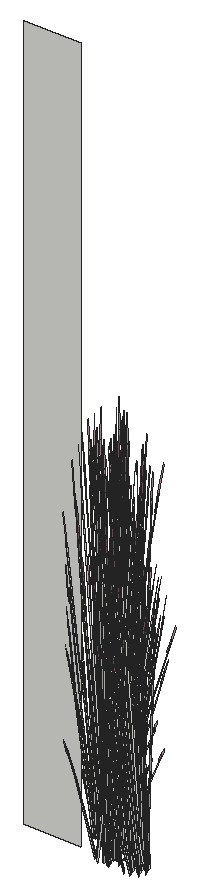
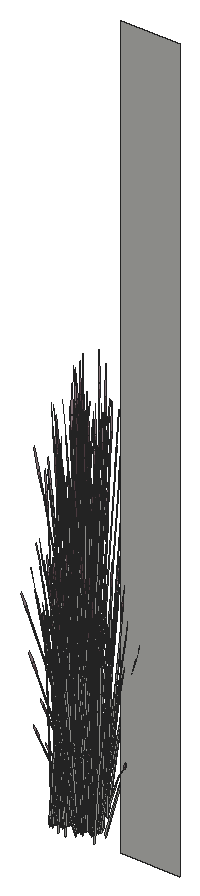
# SketchUp Ruby script. Lengths in inches.
U = 1.inch
M = Sketchup.active_model
def pt(a) = Geom::Point3d.new(a.map { |v| v * U })
def face(e, loops, mat)
  f = e.add_face(loops[0].map { |a| pt(a) })
  loops[1..].each { |l| e.add_face(l.map { |a| pt(a) }).erase! }
  f.material = f.back_material = mat if mat
  f
end
# faces: each face lists its corners as indices into pts; further lists are holes
def faces(e, pts, list, mat = nil) = list.each { |f| face(e, (f[0].is_a?(Array) ? f : [f]).map { |l| l.map { |i| pts[i] } }, mat) }
# xy, xz, yz: faces in a plane at the given z, y or x. An outline is a flat list of corners, or four numbers for a rectangle; further outlines are holes
def ring(l) = l.size == 4 ? [[l[0], l[1]], [l[2], l[1]], [l[2], l[3]], [l[0], l[3]]] : l.each_slice(2).to_a
def flat(e, list, mat, &to3) = list.each { |f| face(e, (f[0].is_a?(Array) ? f : [f]).map { |l| ring(l).map { |u, v| to3.(u, v) } }, mat) }
def xy(e, z, list, mat = nil) = flat(e, list, mat) { |x, y| [x, y, z] }
def xz(e, y, list, mat = nil) = flat(e, list, mat) { |x, z| [x, y, z] }
def yz(e, x, list, mat = nil) = flat(e, list, mat) { |y, z| [x, y, z] }
def lines(e, pts, list) = list.each { |a, b| e.add_line(pt(pts[a]), pt(pts[b])) }
# prism: a flat outline (further loops are holes) pulled along v
def prism(e, loops, v, mat = nil)
  f = face(e, loops, mat); d = Geom::Vector3d.new(v.map { |x| x * U })
  f.pushpull(f.normal.samedirection?(d) ? d.length : -d.length)
end
def box(e, o, s, mat = nil) = prism(e, [[o, [o[0] + s[0], o[1], o[2]], [o[0] + s[0], o[1] + s[1], o[2]], [o[0], o[1] + s[1], o[2]]]], [0, 0, s[2]], mat)
def at(x, y, z, deg = 0) = Geom::Transformation.translation(pt([x, y, z])) * Geom::Transformation.rotation(ORIGIN, Z_AXIS, deg.degrees)
def axes(o, x, y, z) = Geom::Transformation.new([*x, 0, *y, 0, *z, 0, *pt(o).to_a, 1])
def part(name) = M.definitions.add(name)
# library, detail: a bought-in or finely detailed component or shape, given as its bounding box
def library(name, o, s) = part(name).tap { |d| box(d.entities, o, s) }
def detail(e, o, s) = box(e.add_group.entities, o, s)
def put(e, d, t, mat = nil) = e.add_instance(d, t).tap { |i| i.material = mat if mat }
def group(e, t, mat = nil) = e.add_group.tap { |g| g.transformation = t; g.material = mat if mat }.entities
root = M.entities
M.materials.add("LightPink_Translucent").color = [144, 107, 117]
M.materials["LightPink_Translucent"].alpha = 0.75
c1 = part("blade")
p = [[2.15,0.21,22],[0,0.17,0],[0.09,0.45,0],[2.18,0.31,22],[2.29,0.31,22],[0.38,0.45,0],
  [2.48,0.24,33],[2.49,0.24,33],[2.48,0.22,33]]
faces(c1.entities,p,[[0,1,2,3],[4,5,2,3],[6,3,4,7],[8,0,3,6]])
c2 = part("seeds")
p = [[0.3,-0.1,1.38],[-0.01,-0.03,1.59],[-0.01,-0.03,0.03],[0.14,-0.07,-0.07],[0.29,-0.03,3],[0.15,0.01,3.11]]
faces(c2.entities,p,[[0,1,2,3],[1,0,4,5]],"LightPink_Translucent")
c3 = part("blade with seeds")
put(c3.entities,c1,at(0,0,0))
put(c3.entities,c2,axes([2.4,0.25,30.99],[1.5799,-0.05474,1.17369],[-0.12525,1.92788,0.29478],[-0.07173,-0.02425,1.56792]))
xz(root,652.9,[[321.57,621,330.57,735]])
put(root,c3,axes([334.34,651.43,623.6],[0.12246,-0.09864,1.71376],[0.1031,0.45582,0.13857],[-0.19225,0.10302,0.73262]))
put(root,c3,axes([333.96,652.2,622.31],[0.12266,0.03828,1.43002],[0.07906,0.39104,-0.30754],[-0.16661,0.0732,0.61141]))
put(root,c3,axes([335.04,650.95,623.07],[0.10032,-0.06746,1.77064],[0.0346,0.47103,0.13857],[-0.2173,0.0625,0.63284]))
put(root,c3,axes([333.96,651.27,624.4375],[-0.05763,0.06055,1.74944],[0.0049,0.44239,-0.27667],[-0.13211,0.05753,0.14031]))
put(root,c3,axes([334.15,651.01,624.25],[-0.29332,-0.1301,-0.35414],[0.08555,-0.37955,0.4572],[-0.11809,0.0348,0.87481]))
put(root,c3,axes([333.32,651.71,624.43],[0.04504,0.01251,1.77383],[0.13934,0.41205,-0.16761],[-0.0922,0.10815,0.31391]))
put(root,c3,axes([334.35,651.21,624.4],[-0.09562,0.42421,-0.51099],[-0.32782,-0.1454,-0.3958],[-0.13199,0.0389,0.97773]))
put(root,c3,axes([334.18,651.18,621.22],[0.00895,0.0735,1.76342],[-0.18044,0.38382,-0.26939],[-0.12817,-0.01935,0.30037]))
put(root,c3,axes([333.7,653.02,622.49],[0.14709,-0.21136,1.1486],[0.05804,0.3346,0.84392],[-0.1063,0.05991,0.25299]))
put(root,c3,axes([334.22,650.97,624.46],[0.09971,-0.42522,0.48003],[0.32782,0.1454,0.3958],[-0.12892,0.02555,0.9933]))
put(root,c3,axes([334.33,650.84,624.76],[0.17758,0.42229,-0.1216],[-0.31518,0.20752,-0.67495],[-0.13282,0.05572,1.02557]))
put(root,c3,axes([334.19,650.85,624.45],[-0.12963,-0.31798,0.0643],[0.23638,-0.15564,0.50621],[-0.1042,0.03071,0.77189]))
put(root,c3,axes([334.78,651.73,623.6],[0.08815,-0.14329,1.71376],[0.22258,0.38678,0.13857],[-0.15267,0.17614,0.73262]))
put(root,c3,axes([334.25,652.11,624.25],[-0.30722,0.06665,-0.35414],[-0.08112,-0.381,0.4572],[-0.08804,0.10234,0.87481]))
put(root,c3,axes([334.09,653.24,621.22],[0.04734,0.04659,1.76342],[0.08027,0.4317,-0.26939],[-0.10492,0.09206,0.30037]))
put(root,c3,axes([334.29,652.03,624.46],[-0.08753,-0.42921,0.48003],[0.34336,-0.07449,0.3958],[-0.1012,0.10094,0.9933]))
put(root,c3,axes([334.23,651.94,624.45],[-0.2423,-0.19613,0.0643],[0.14107,-0.2793,0.50621],[-0.07768,0.0903,0.77189]))
put(root,c3,axes([334.72,652.09,623.6],[0.06572,-0.16029,1.71376],[0.27569,0.33172,0.13857],[-0.12437,0.20675,0.73262]))
put(root,c3,axes([334.46,650.97,624.78],[0.29332,0.1301,0.35414],[-0.08555,0.37955,-0.4572],[-0.11809,0.0348,0.87481]))
put(root,c3,axes([334.51,652.15,624.4],[0.09067,0.42583,-0.51099],[-0.34336,0.07449,-0.3958],[-0.0984,0.11438,0.97773]))
put(root,c3,axes([335.36,651.85,621.78],[-0.36714,-0.07646,-0.62353],[0.07747,-0.47163,-0.16365],[-0.10956,-0.05715,1.37633]))
put(root,c3,axes([334.88,652.74,621.74],[-0.33032,-0.23318,-0.49651],[0.19744,-0.41812,0],[-0.07523,-0.05311,1.57504]))
put(root,c3,axes([334.35,651.85,624.76],[0.32648,0.25715,-0.1216],[-0.18809,0.3724,-0.67495],[-0.09224,0.12945,1.02557]))
put(root,c3,axes([335.08,653.02,622.1],[-0.22066,0.46731,0],[-0.36918,-0.26061,-0.51607],[-0.08408,-0.05936,1.63711]))
put(root,c3,axes([333.81,652.96,625.37],[0.31145,0.12449,-0.06488],[-0.0958,0.38314,-0.29416],[-0.05094,0.05817,0.97024]))
put(root,c3,axes([334.5,651.88,624.78],[0.30722,-0.06665,0.35414],[0.08112,0.381,-0.4572],[-0.08804,0.10234,0.87481]))
put(root,c3,axes([335.78,651.92,622.39],[-0.35635,0.30962,-0.29095],[-0.23697,-0.43749,-0.50002],[-0.08792,-0.04443,1.59708]))
put(root,c3,axes([334.8,652.89,624.46],[-0.25132,-0.3182,0.48003],[0.2669,-0.27442,0.3958],[-0.04636,0.14929,0.9933]))
put(root,c3,axes([334.97,652.57,621.75],[-0.08291,-0.40636,-0.30978],[0.32928,-0.11539,0.30978],[-0.06638,-0.04686,1.38974]))
put(root,c3,axes([334.7,652.86,624.45],[-0.29004,-0.02173,0.0643],[0.00795,-0.32812,0.50621],[-0.03035,0.12569,0.77189]))
put(root,c3,axes([336.02,652.25,621.78],[-0.23773,0.35053,-0.62353],[-0.29532,-0.31785,-0.16365],[-0.09526,0.08744,1.37633]))
put(root,c3,axes([336.18,652.06,622.1875],[-0.34464,-0.37536,-0.25192],[0.29,-0.42149,0.5513],[-0.0928,0.04391,1.68216]))
put(root,c3,axes([336.01,651.98,621.93],[-0.38326,0.02879,-0.44739],[-0.03466,-0.47788,0.21531],[-0.06861,0.04843,1.43643]))
put(root,c3,axes([335.27,652.78,622.2],[0.33032,0.23318,0.49651],[-0.19744,0.41812,0],[-0.07523,-0.05311,1.57504]))
put(root,c3,axes([335.75,652.05,622.34],[-0.06809,0.4162,0.1448],[-0.33266,-0.07225,-0.41347],[-0.06054,-0.04274,1.26744]))
put(root,c3,axes([336.41,653.21,621.74],[-0.33032,0.23318,-0.49651],[-0.19744,-0.41812,0],[-0.07523,0.05311,1.57504]))
put(root,c3,axes([336.43,653.09,621.92],[-0.21791,-0.46895,-0.05142],[0.36918,-0.26061,0.51607],[-0.09097,0.04465,1.6363]))
put(root,c3,axes([336.33,653.03,621.75],[-0.32928,-0.11539,-0.30978],[0.08291,-0.40636,0.30978],[-0.06638,0.04686,1.38974]))
put(root,c3,axes([334.92,652.64,624.78],[0.23881,-0.24554,0.35414],[0.22606,0.28036,-0.4572],[-0.0344,0.14245,0.87481]))
put(root,c3,axes([336.52,651.29,622.57],[-0.00964,-0.43909,1.41272],[0.43635,0.11382,0.59816],[-0.1032,0.24027,1.3335]))
put(root,c3,axes([336.27,651.85,622.39],[0.04113,0.53214,-0.29095],[-0.42835,0.03218,-0.50002],[-0.07543,0.07088,1.59708]))
put(root,c3,axes([335.64,651.66,622.09],[0.44609,0.09826,0.45755],[-0.09078,0.55493,0.17955],[-0.06519,-0.05359,1.58856]))
put(root,c3,axes([335.52,651.55,622.44],[-0.17124,0.42022,0.44739],[-0.35581,-0.20224,-0.21531],[0,-0.09687,1.43643]))
put(root,c3,axes([335.4,652.54,622.2],[0.37926,-0.12378,0.17642],[0.09365,0.46065,0.35086],[-0.03382,-0.06712,1.60407]))
put(root,c3,axes([335.89,652.61,621.92],[-0.35581,-0.20937,0],[0.17124,-0.43505,0],[0,0,1.62707]))
put(root,c3,axes([336.71,653.14,622.1],[0.22066,0.46731,0],[-0.36918,0.26061,-0.51607],[-0.08408,0.05936,1.63711]))
put(root,c3,axes([338.8,651.43,623.1],[0.12246,-0.09864,1.71376],[0.1031,0.45582,0.13857],[-0.19225,0.10302,0.73262]))
put(root,c3,axes([336.53,652.57,622.2],[0.10196,-0.46348,0.17642],[0.3731,0.13116,0.35086],[-0.06445,0.00226,1.60407]))
put(root,c3,axes([336.35,651.95,622.34],[0.26075,0.2802,0.1448],[-0.2175,0.31612,-0.41347],[-0.06054,0.04274,1.26744]))
put(root,c3,axes([338.42,652.2,621.81],[0.12266,0.03828,1.43002],[0.07906,0.39104,-0.30754],[-0.16661,0.0732,0.61141]))
put(root,c3,axes([336.26,651.61,622.02],[-0.32829,-0.4014,-0.06131],[0.32849,-0.40164,0],[-0.01146,-0.01402,1.75571]))
put(root,c3,axes([336.35,651.75,622.44],[0.38326,-0.02879,0.44739],[0.03466,0.47788,-0.21531],[-0.06861,0.04843,1.43643]))
put(root,c3,axes([339.5,650.95,622.57],[0.10032,-0.06746,1.77064],[0.0346,0.47103,0.13857],[-0.2173,0.0625,0.63284]))
put(root,c3,axes([336.44,652.85,622.05],[0.44186,0.15158,0.30756],[-0.11054,0.54181,-0.36492],[-0.07313,0.06781,1.64885]))
put(root,c3,axes([336.63,652.82,622.2],[0.33032,-0.23318,0.49651],[0.19744,0.41812,0],[-0.07523,0.05311,1.57504]))
put(root,c3,axes([335.97,652.43,621.93],[-0.11516,-0.40207,0],[0.32884,-0.1408,0],[0,0,1.54371]))
put(root,c3,axes([338.42,651.27,623.9375],[-0.05763,0.06055,1.74944],[0.0049,0.44239,-0.27667],[-0.13211,0.05753,0.14031]))
put(root,c3,axes([338.61,651.01,623.75],[-0.29332,-0.1301,-0.35414],[0.08555,-0.37955,0.4572],[-0.11809,0.0348,0.87481]))
put(root,c3,axes([336.43,651.64,621.93],[-0.17124,0.42022,-0.44739],[-0.35581,-0.20224,0.21531],[0,0.09687,1.43643]))
put(root,c3,axes([337.78,651.71,623.93],[0.04504,0.01251,1.77383],[0.13934,0.41205,-0.16761],[-0.0922,0.10815,0.31391]))
put(root,c3,axes([337.11,651.38,622.2],[-0.2773,-0.3397,0.17642],[0.27945,-0.32949,0.35086],[-0.03063,0.06937,1.60407]))
put(root,c3,axes([338.81,651.21,623.9],[-0.09562,0.42421,-0.51099],[-0.32782,-0.1454,-0.3958],[-0.13199,0.0389,0.97773]))
put(root,c3,axes([336.15,651.1875,621.93],[0,-0.53961,0],[0.44133,0,0],[0,0,1.79456]))
put(root,c3,axes([336.37,651.4,622.02],[0,0.53934,-0.05637],[-0.44133,0,0],[0,0.01695,1.79368]))
put(root,c3,axes([338.64,651.18,620.72],[0.00895,0.0735,1.76342],[-0.18044,0.38382,-0.26939],[-0.12817,-0.01935,0.30037]))
put(root,c3,axes([335.59,653.05,624.78],[0.1064,-0.35863,0.35414],[0.31043,0.1046,-0.4572],[0.02846,0.14439,0.87481]))
put(root,c3,axes([335.43,650.15,622.2],[-0.10196,0.46348,0.17642],[-0.3731,-0.13116,0.35086],[0.06445,-0.00226,1.60407]))
put(root,c3,axes([336.16,652.45,622.02],[0.15345,0.53576,-0.06012],[-0.43845,0.18773,0],[0.00536,0.01871,1.72173]))
put(root,c3,axes([338.16,653.02,621.99],[0.14709,-0.21136,1.1486],[0.05804,0.3346,0.84392],[-0.1063,0.05991,0.25299]))
put(root,c3,axes([337.43,651.74,621.92],[-0.44111,-0.00373,-0.04976],[0,-0.52122,0.49943],[-0.01386,0.11865,1.58352]))
put(root,c3,axes([338.68,650.97,623.96],[0.09971,-0.42522,0.48003],[0.32782,0.1454,0.3958],[-0.12892,0.02555,0.9933]))
put(root,c3,axes([338.79,650.84,624.26],[0.17758,0.42229,-0.1216],[-0.31518,0.20752,-0.67495],[-0.13282,0.05572,1.02557]))
put(root,c3,axes([339.875,651.43,623.19],[0.12246,-0.09864,1.71376],[0.1031,0.45582,0.13857],[-0.19225,0.10302,0.73262]))
put(root,c3,axes([336.5625,650.18,622.2],[-0.37926,0.12378,0.17642],[-0.09365,-0.46065,0.35086],[0.03382,0.06712,1.60407]))
put(root,c3,axes([338.65,650.85,623.95],[-0.12963,-0.31798,0.0643],[0.23638,-0.15564,0.50621],[-0.1042,0.03071,0.77189]))
put(root,c3,axes([339.25,651.73,623.1],[0.08815,-0.14329,1.71376],[0.22258,0.38678,0.13857],[-0.15267,0.17614,0.73262]))
put(root,c3,axes([338.71,652.11,623.75],[-0.30722,0.06665,-0.35414],[-0.08112,-0.381,0.4572],[-0.08804,0.10234,0.87481]))
put(root,c3,axes([339.49,652.2,621.91],[0.12266,0.03828,1.43002],[0.07906,0.39104,-0.30754],[-0.16661,0.0732,0.61141]))
put(root,c3,axes([336.01,654.32,625.37],[0.2439,-0.26754,-0.06488],[0.22348,0.29302,-0.29416],[0.01573,0.08303,0.97024]))
put(root,c3,axes([335.94,650.85,622.09],[-0.29264,0.42323,0.45755],[-0.34767,-0.3736,0.17955],[0.07055,-0.04224,1.58856]))
put(root,c3,axes([338.55,653.24,620.72],[0.04734,0.04659,1.76342],[0.08027,0.4317,-0.26939],[-0.10492,0.09206,0.30037]))
put(root,c3,axes([336.44,651.52,621.9375],[0.24637,0.30123,0],[-0.24637,0.30123,0],[0,0,1.69266]))
put(root,c3,axes([336.4375,651.16,622.44],[0.17124,-0.42022,0.44739],[0.35581,0.20224,-0.21531],[0,0.09687,1.43643]))
put(root,c3,axes([336.29,652.62,621.93],[0.35581,0.20937,0],[-0.17124,0.43505,0],[0,0,1.74954]))
put(root,c3,axes([340.58,650.95,622.66],[0.10032,-0.06746,1.77064],[0.0346,0.47103,0.13857],[-0.2173,0.0625,0.63284]))
put(root,c3,axes([338.75,652.03,623.96],[-0.08753,-0.42921,0.48003],[0.34336,-0.07449,0.3958],[-0.1012,0.10094,0.9933]))
put(root,c3,axes([336.32,651.0625,622.11],[-0.44609,-0.09826,0.49198],[0.09078,-0.55493,0.19306],[0.06519,0.05359,1.70813]))
put(root,c3,axes([337.34,651.82,621.75],[-0.24637,0.29097,-0.30978],[-0.24637,-0.29097,0.30978],[0,0.09372,1.38974]))
put(root,c3,axes([338.6875,651.94,623.95],[-0.2423,-0.19613,0.0643],[0.14107,-0.2793,0.50621],[-0.07768,0.0903,0.77189]))
put(root,c3,axes([336.63,651.77,621.82],[0.12941,0.42699,-0.69212],[-0.37279,0.15378,-0.18165],[0.0143,0.14459,1.52773]))
put(root,c3,axes([336.45,651.31,621.93],[0.39487,0,0],[0,0.48281,0],[0,0,1.78407]))
put(root,c3,axes([339.5,651.27,624.03],[-0.05763,0.06055,1.74944],[0.0049,0.44239,-0.27667],[-0.13211,0.05753,0.14031]))
put(root,c3,axes([336.07,650.78,622.44],[-0.21202,-0.39143,0.44739],[0.32115,-0.27564,-0.21531],[0.06861,0.04843,1.43643]))
put(root,c3,axes([339.18,652.09,623.1],[0.06572,-0.16029,1.71376],[0.27569,0.33172,0.13857],[-0.12437,0.20675,0.73262]))
put(root,c3,axes([336.59,651.26,622.34],[0.32884,-0.136,0.1448],[0.11516,0.38837,-0.41347],[0,0.08547,1.26744]))
put(root,c3,axes([339.69,651.01,623.84],[-0.29332,-0.1301,-0.35414],[0.08555,-0.37955,0.4572],[-0.11809,0.0348,0.87481]))
put(root,c3,axes([338.92,650.97,624.28],[0.29332,0.1301,0.35414],[-0.08555,0.37955,-0.4572],[-0.11809,0.0348,0.87481]))
put(root,c3,axes([336.47,651.29,622.39],[0.39748,0.22252,-0.29095],[-0.19139,0.46966,-0.50002],[0.01249,0.11531,1.59708]))
put(root,c3,axes([338.97,652.15,623.9],[0.09067,0.42583,-0.51099],[-0.34336,0.07449,-0.3958],[-0.0984,0.11438,0.97773]))
put(root,c3,axes([338.86,651.71,624.03],[0.04504,0.01251,1.77383],[0.13934,0.41205,-0.16761],[-0.0922,0.10815,0.31391]))
put(root,c3,axes([339.89,651.21,624],[-0.09562,0.42421,-0.51099],[-0.32782,-0.1454,-0.3958],[-0.13199,0.0389,0.97773]))
put(root,c3,axes([339.82,651.85,621.28],[-0.36714,-0.07646,-0.62353],[0.07747,-0.47163,-0.16365],[-0.10956,-0.05715,1.37633]))
put(root,c3,axes([339.72,651.18,620.81],[0.00895,0.0735,1.76342],[-0.18044,0.38382,-0.26939],[-0.12817,-0.01935,0.30037]))
put(root,c3,axes([337.34,651.4,622.2],[0,-0.46636,0.49651],[0.39487,0,0],[0,0.10622,1.57504]))
put(root,c3,axes([337.51,651.83,621.74],[0,0.46636,-0.49651],[-0.39487,0,0],[0,0.10622,1.57504]))
put(root,c3,axes([336.45,653.24,624.46],[-0.35104,0.10702,0.48003],[-0.06092,-0.41983,0.3958],[0.08256,0.12373,0.9933]))
put(root,c3,axes([336.38,653.33,624.45],[-0.16041,0.29625,0.0643],[-0.22843,-0.17248,0.50621],[0.07385,0.09498,0.77189]))
put(root,c3,axes([336.21,650.67,622.34],[0.06809,-0.4162,0.1448],[0.33266,0.07225,-0.41347],[0.06054,0.04274,1.26744]))
put(root,c3,axes([339.24,653.02,622.08],[0.14709,-0.21136,1.1486],[0.05804,0.3346,0.84392],[-0.1063,0.05991,0.25299]))
put(root,c3,axes([339.34,652.74,621.24],[-0.33032,-0.23318,-0.49651],[0.19744,-0.41812,0],[-0.07523,-0.05311,1.57504]))
put(root,c3,axes([338.81,651.85,624.26],[0.32648,0.25715,-0.1216],[-0.18809,0.3724,-0.67495],[-0.09224,0.12945,1.02557]))
put(root,c3,axes([336.69,649.94,622.2],[-0.33032,-0.23318,0.49651],[0.19744,-0.41812,0],[0.07523,0.05311,1.57504]))
put(root,c3,axes([339.54,653.02,621.6],[-0.22066,0.46731,0],[-0.36918,-0.26061,-0.51607],[-0.08408,-0.05936,1.63711]))
put(root,c3,axes([339.75,650.97,624.05],[0.09971,-0.42522,0.48003],[0.32782,0.1454,0.3958],[-0.12892,0.02555,0.9933]))
put(root,c3,axes([339.87,650.84,624.35],[0.17758,0.42229,-0.1216],[-0.31518,0.20752,-0.67495],[-0.13282,0.05572,1.02557]))
put(root,c3,axes([336.4,652.375,621.91],[0.37054,-0.15823,-0.19198],[0.1302,0.45581,0.00008],[0.0409,-0.01749,1.73897]))
put(root,c3,axes([339.73,650.85,624.05],[-0.12963,-0.31798,0.0643],[0.23638,-0.15564,0.50621],[-0.1042,0.03071,0.77189]))
put(root,c3,axes([340.32,651.73,623.19],[0.08815,-0.14329,1.71376],[0.22258,0.38678,0.13857],[-0.15267,0.17614,0.73262]))
put(root,c3,axes([339.79,652.11,623.84],[-0.30722,0.06665,-0.35414],[-0.08112,-0.381,0.4572],[-0.08804,0.10234,0.87481]))
put(root,c3,axes([338.27,652.96,624.87],[0.31145,0.12449,-0.06488],[-0.0958,0.38314,-0.29416],[-0.05094,0.05817,0.97024]))
put(root,c3,axes([339.625,653.24,620.81],[0.04734,0.04659,1.76342],[0.08027,0.4317,-0.26939],[-0.10492,0.09206,0.30037]))
put(root,c3,axes([338.97,651.88,624.28],[0.30722,-0.06665,0.35414],[0.08112,0.381,-0.4572],[-0.08804,0.10234,0.87481]))
put(root,c3,axes([336.33,652.99,624.78],[-0.05451,-0.37564,0.35414],[0.31161,-0.09919,-0.4572],[0.0837,0.10765,0.87481]))
put(root,c3,axes([336.4,651.02,621.93],[0.21202,0.39143,-0.44739],[-0.32115,0.27564,0.21531],[0.06861,0.04843,1.43643]))
put(root,c3,axes([341.21,651.43,623.58],[0.12246,-0.09864,1.71376],[0.1031,0.45582,0.13857],[-0.19225,0.10302,0.73262]))
put(root,c3,axes([339.83,652.03,624.05],[-0.08753,-0.42921,0.48003],[0.34336,-0.07449,0.3958],[-0.1012,0.10094,0.9933]))
put(root,c3,axes([336.54,650.82,624.2],[-0.30498,-0.24231,1.38283],[0.32203,-0.37727,0.59665],[0.0984,0.22736,1.33663]))
put(root,c3,axes([336.03,653.51,624.43],[0.00104,-0.05646,1.77383],[0.30246,-0.2491,-0.16761],[0.10506,0.08891,0.31391]))
put(root,c3,axes([340.83,652.2,622.3],[0.12266,0.03828,1.43002],[0.07906,0.39104,-0.30754],[-0.16661,0.0732,0.61141]))
put(root,c3,axes([337,652.8,622.49],[-0.19872,-0.13409,1.1486],[0.2566,-0.13625,0.84392],[0.06921,0.11541,0.25299]))
put(root,c3,axes([336.3,652.65,622.31],[0.00623,-0.15459,1.43002],[0.29764,-0.17268,-0.30754],[0.09188,0.18503,0.61141]))
put(root,c3,axes([339.76,651.94,624.05],[-0.2423,-0.19613,0.0643],[0.14107,-0.2793,0.50621],[-0.07768,0.0903,0.77189]))
put(root,c3,axes([340.24,651.92,621.89],[-0.35635,0.30962,-0.29095],[-0.23697,-0.43749,-0.50002],[-0.08792,-0.04443,1.59708]))
put(root,c3,axes([339.26,652.89,623.96],[-0.25132,-0.3182,0.48003],[0.2669,-0.27442,0.3958],[-0.04636,0.14929,0.9933]))
put(root,c3,axes([341.91,650.95,623.05],[0.10032,-0.06746,1.77064],[0.0346,0.47103,0.13857],[-0.2173,0.0625,0.63284]))
put(root,c3,axes([340.26,652.09,623.19],[0.06572,-0.16029,1.71376],[0.27569,0.33172,0.13857],[-0.12437,0.20675,0.73262]))
put(root,c3,axes([339.43,652.57,621.25],[-0.08291,-0.40636,-0.30978],[0.32928,-0.11539,0.30978],[-0.06638,-0.04686,1.38974]))
put(root,c3,axes([339.16,652.86,623.95],[-0.29004,-0.02173,0.0643],[0.00795,-0.32812,0.50621],[-0.03035,0.12569,0.77189]))
put(root,c3,axes([336.98,650.15,621.75],[0.08291,0.40636,-0.30978],[-0.32928,0.11539,0.30978],[0.06638,0.04686,1.38974]))
put(root,c3,axes([337.6,651.48,622.1],[0.44133,0,0],[0,0.52122,-0.51607],[0,0.11871,1.63711]))
put(root,c3,axes([339.99,650.97,624.37],[0.29332,0.1301,0.35414],[-0.08555,0.37955,-0.4572],[-0.11809,0.0348,0.87481]))
put(root,c3,axes([340.05,652.15,624],[0.09067,0.42583,-0.51099],[-0.34336,0.07449,-0.3958],[-0.0984,0.11438,0.97773]))
put(root,c3,axes([336.18,650.8,622.39],[0.35635,-0.30962,-0.29095],[0.23697,0.43749,-0.50002],[0.08792,0.04443,1.59708]))
put(root,c3,axes([340.48,652.25,621.28],[-0.23773,0.35053,-0.62353],[-0.29532,-0.31785,-0.16365],[-0.09526,0.08744,1.37633]))
put(root,c3,axes([337.04,653.41,622.39],[-0.22633,-0.01463,1.0506],[0.14947,-0.31064,0.58006],[0.08941,0.11036,0.8241]))
put(root,c3,axes([340.84,651.27,624.42],[-0.05763,0.06055,1.74944],[0.0049,0.44239,-0.27667],[-0.13211,0.05753,0.14031]))
put(root,c3,axes([340.9,651.85,621.375],[-0.36714,-0.07646,-0.62353],[0.07747,-0.47163,-0.16365],[-0.10956,-0.05715,1.37633]))
put(root,c3,axes([341.02,651.01,624.23],[-0.29332,-0.1301,-0.35414],[0.08555,-0.37955,0.4572],[-0.11809,0.0348,0.87481]))
put(root,c3,axes([340.64,652.06,621.6875],[-0.34464,-0.37536,-0.25192],[0.29,-0.42149,0.5513],[-0.0928,0.04391,1.68216]))
put(root,c3,axes([336.31,653.18,624.76],[0.21031,-0.39918,-0.1216],[0.30457,0.22997,-0.67495],[0.10587,0.11278,1.02557]))
put(root,c3,axes([335.28,650.53,621.32],[-0.3474,0.18671,1.28929],[-0.11057,-0.53572,0.50096],[0.21332,0.00891,1.46642]))
put(root,c3,axes([340.19,651.71,624.42],[0.04504,0.01251,1.77383],[0.13934,0.41205,-0.16761],[-0.0922,0.10815,0.31391]))
put(root,c3,axes([340.42,652.74,621.33],[-0.33032,-0.23318,-0.49651],[0.19744,-0.41812,0],[-0.07523,-0.05311,1.57504]))
put(root,c3,axes([341.22,651.21,624.39],[-0.09562,0.42421,-0.51099],[-0.32782,-0.1454,-0.3958],[-0.13199,0.0389,0.97773]))
put(root,c3,axes([339.88,651.85,624.35],[0.32648,0.25715,-0.1216],[-0.18809,0.3724,-0.67495],[-0.09224,0.12945,1.02557]))
put(root,c3,axes([340.47,651.98,621.43],[-0.38326,0.02879,-0.44739],[-0.03466,-0.47788,0.21531],[-0.06861,0.04843,1.43643]))
put(root,c3,axes([340.62,653.02,621.69],[-0.22066,0.46731,0],[-0.36918,-0.26061,-0.51607],[-0.08408,-0.05936,1.63711]))
put(root,c3,axes([341.06,651.18,621.2],[0.00895,0.0735,1.76342],[-0.18044,0.38382,-0.26939],[-0.12817,-0.01935,0.30037]))
put(root,c3,axes([336.56,652.98,624.4],[0.34827,-0.11086,-0.51099],[0.06092,0.41983,-0.3958],[0.09354,0.12031,0.97773]))
put(root,c3,axes([339.73,652.78,621.7],[0.33032,0.23318,0.49651],[-0.19744,0.41812,0],[-0.07523,-0.05311,1.57504]))
put(root,c3,axes([336.96,652.48,624.78],[-0.20082,-0.29199,0.35414],[0.2293,-0.2764,-0.4572],[0.1165,0.04206,0.87481]))
put(root,c3,axes([339.35,652.96,624.96],[0.31145,0.12449,-0.06488],[-0.0958,0.38314,-0.29416],[-0.05094,0.05817,0.97024]))
put(root,c3,axes([340.57,653.02,622.47],[0.14709,-0.21136,1.1486],[0.05804,0.3346,0.84392],[-0.1063,0.05991,0.25299]))
put(root,c3,axes([337.08,649.98,621.74],[0.33032,0.23318,-0.49651],[-0.19744,0.41812,0],[0.07523,0.05311,1.57504]))
put(root,c3,axes([340.04,651.88,624.37],[0.30722,-0.06665,0.35414],[0.08112,0.381,-0.4572],[-0.08804,0.10234,0.87481]))
put(root,c3,axes([337.14,652.74,624.45],[-0.01777,0.35463,0.0643],[-0.26836,-0.00972,0.50621],[0.1028,0.03711,0.77189]))
put(root,c3,axes([337.06,653.3,621.22],[0.02571,-0.06733,1.76342],[0.32373,-0.19829,-0.26939],[0.09815,0.10263,0.30037]))
put(root,c3,axes([340.21,652.05,621.84],[-0.06809,0.4162,0.1448],[-0.33266,-0.07225,-0.41347],[-0.06054,-0.04274,1.26744]))
put(root,c3,axes([337.16,652.63,624.46],[-0.26024,0.30729,0.48003],[-0.22444,-0.32634,0.3958],[0.1221,0.05668,0.9933]))
put(root,c3,axes([341.09,650.97,624.44],[0.09971,-0.42522,0.48003],[0.32782,0.1454,0.3958],[-0.12892,0.02555,0.9933]))
put(root,c3,axes([340.87,653.21,621.24],[-0.33032,0.23318,-0.49651],[-0.19744,-0.41812,0],[-0.07523,0.05311,1.57504]))
put(root,c3,axes([341.21,650.84,624.74],[0.17758,0.42229,-0.1216],[-0.31518,0.20752,-0.67495],[-0.13282,0.05572,1.02557]))
put(root,c3,axes([340.89,653.09,621.42],[-0.21791,-0.46895,-0.05142],[0.36918,-0.26061,0.51607],[-0.09097,0.04465,1.6363]))
put(root,c3,axes([337.84,652.68,623.65],[-0.06755,-0.39203,-0.03492],[0.31928,-0.09013,-0.15832],[0.06667,0.02485,0.52218]))
put(root,c3,axes([337.29,651.66,624.78],[-0.29332,-0.1301,0.35414],[0.08555,-0.37955,-0.4572],[0.11809,-0.0348,0.87481]))
put(root,c3,axes([341.0625,650.85,624.4375],[-0.12963,-0.31798,0.0643],[0.23638,-0.15564,0.50621],[-0.1042,0.03071,0.77189]))
put(root,c3,axes([341.66,651.73,623.58],[0.08815,-0.14329,1.71376],[0.22258,0.38678,0.13857],[-0.15267,0.17614,0.73262]))
put(root,c3,axes([341.13,652.11,624.23],[-0.30722,0.06665,-0.35414],[-0.08112,-0.381,0.4572],[-0.08804,0.10234,0.87481]))
put(root,c3,axes([336.59,650.87,621.78],[0.36714,0.07646,-0.62353],[-0.07747,0.47163,-0.16365],[0.10956,0.05715,1.37633]))
put(root,c3,axes([338.16,651.15,621.99],[-0.21881,-0.29821,-0.06488],[0.23965,-0.27324,-0.29416],[0.0679,-0.01924,0.97024]))
put(root,c3,axes([340.79,653.03,621.25],[-0.32928,-0.11539,-0.30978],[0.08291,-0.40636,0.30978],[-0.06638,0.04686,1.38974]))
put(root,c3,axes([340.96,653.24,621.2],[0.04734,0.04659,1.76342],[0.08027,0.4317,-0.26939],[-0.10492,0.09206,0.30037]))
put(root,c3,axes([339.38,652.64,624.28],[0.23881,-0.24554,0.35414],[0.22606,0.28036,-0.4572],[-0.0344,0.14245,0.87481]))
put(root,c3,axes([341.32,651.92,621.98],[-0.35635,0.30962,-0.29095],[-0.23697,-0.43749,-0.50002],[-0.08792,-0.04443,1.59708]))
put(root,c3,axes([340.33,652.89,624.05],[-0.25132,-0.3182,0.48003],[0.2669,-0.27442,0.3958],[-0.04636,0.14929,0.9933]))
put(root,c3,axes([340.98,651.29,622.07],[-0.00964,-0.43909,1.41272],[0.43635,0.11382,0.59816],[-0.1032,0.24027,1.3335]))
put(root,c3,axes([340.51,652.57,621.35],[-0.08291,-0.40636,-0.30978],[0.32928,-0.11539,0.30978],[-0.06638,-0.04686,1.38974]))
put(root,c3,axes([340.24,652.86,624.05],[-0.29004,-0.02173,0.0643],[0.00795,-0.32812,0.50621],[-0.03035,0.12569,0.77189]))
put(root,c3,axes([341.17,652.03,624.44],[-0.08753,-0.42921,0.48003],[0.34336,-0.07449,0.3958],[-0.1012,0.10094,0.9933]))
put(root,c3,axes([340.73,651.85,621.89],[0.04113,0.53214,-0.29095],[-0.42835,0.03218,-0.50002],[-0.07543,0.07088,1.59708]))
put(root,c3,axes([341.1,651.94,624.4375],[-0.2423,-0.19613,0.0643],[0.14107,-0.2793,0.50621],[-0.07768,0.0903,0.77189]))
put(root,c3,axes([341.56,652.25,621.375],[-0.23773,0.35053,-0.62353],[-0.29532,-0.31785,-0.16365],[-0.09526,0.08744,1.37633]))
put(root,c3,axes([336.52,651.88,623.6],[-0.1311,-0.08035,1.71376],[0.27131,-0.33708,0.13857],[0.16909,0.15206,0.73262]))
put(root,c3,axes([341.59,652.09,623.58],[0.06572,-0.16029,1.71376],[0.27569,0.33172,0.13857],[-0.12437,0.20675,0.73262]))
